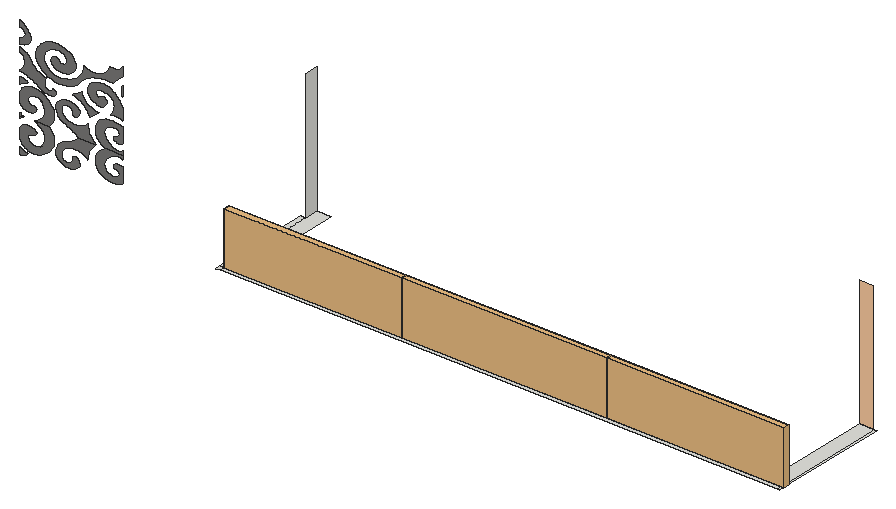
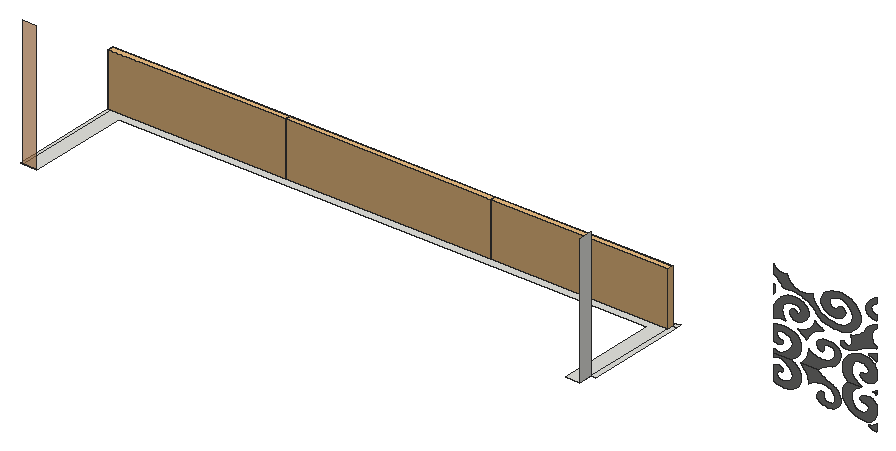
# SketchUp Ruby script. Lengths in inches.
U = 1.inch
M = Sketchup.active_model
def pt(a) = Geom::Point3d.new(a.map { |v| v * U })
def face(e, loops, mat)
  f = e.add_face(loops[0].map { |a| pt(a) })
  loops[1..].each { |l| e.add_face(l.map { |a| pt(a) }).erase! }
  f.material = f.back_material = mat if mat
  f
end
# faces: each face lists its corners as indices into pts; further lists are holes
def faces(e, pts, list, mat = nil) = list.each { |f| face(e, (f[0].is_a?(Array) ? f : [f]).map { |l| l.map { |i| pts[i] } }, mat) }
# xy, xz, yz: faces in a plane at the given z, y or x. An outline is a flat list of corners, or four numbers for a rectangle; further outlines are holes
def ring(l) = l.size == 4 ? [[l[0], l[1]], [l[2], l[1]], [l[2], l[3]], [l[0], l[3]]] : l.each_slice(2).to_a
def flat(e, list, mat, &to3) = list.each { |f| face(e, (f[0].is_a?(Array) ? f : [f]).map { |l| ring(l).map { |u, v| to3.(u, v) } }, mat) }
def xy(e, z, list, mat = nil) = flat(e, list, mat) { |x, y| [x, y, z] }
def xz(e, y, list, mat = nil) = flat(e, list, mat) { |x, z| [x, y, z] }
def yz(e, x, list, mat = nil) = flat(e, list, mat) { |y, z| [x, y, z] }
def lines(e, pts, list) = list.each { |a, b| e.add_line(pt(pts[a]), pt(pts[b])) }
# prism: a flat outline (further loops are holes) pulled along v
def prism(e, loops, v, mat = nil)
  f = face(e, loops, mat); d = Geom::Vector3d.new(v.map { |x| x * U })
  f.pushpull(f.normal.samedirection?(d) ? d.length : -d.length)
end
def box(e, o, s, mat = nil) = prism(e, [[o, [o[0] + s[0], o[1], o[2]], [o[0] + s[0], o[1] + s[1], o[2]], [o[0], o[1] + s[1], o[2]]]], [0, 0, s[2]], mat)
def at(x, y, z, deg = 0) = Geom::Transformation.translation(pt([x, y, z])) * Geom::Transformation.rotation(ORIGIN, Z_AXIS, deg.degrees)
def axes(o, x, y, z) = Geom::Transformation.new([*x, 0, *y, 0, *z, 0, *pt(o).to_a, 1])
def part(name) = M.definitions.add(name)
# library, detail: a bought-in or finely detailed component or shape, given as its bounding box
def library(name, o, s) = part(name).tap { |d| box(d.entities, o, s) }
def detail(e, o, s) = box(e.add_group.entities, o, s)
def put(e, d, t, mat = nil) = e.add_instance(d, t).tap { |i| i.material = mat if mat }
def group(e, t, mat = nil) = e.add_group.tap { |g| g.transformation = t; g.material = mat if mat }.entities
root = M.entities
M.materials.add("[0043_SaddleBrown]4").color = [124, 123, 122]
M.materials.add("[Granite Light Gray]").color = [149, 148, 144]
M.materials.add("[Wood Floor]").color = [224, 152, 88]
M.materials["[Wood Floor]"].alpha = 0.68
c1 = library("Glass Railing",[0,0,0],[139.5,4.76,42])
xy(root,293,[[4300.2,556.4375,4303.63,559.875],[4303.63,556.4375,4742.06,559.875],[4742.06,556.4375,4744,559.875],[4300.2,559.875,4303.63,640.11],[4303.63,559.875,4742.06,559.875,4742.06,651.03,4730.74,651.03,4730.74,571.2,4314.96,571.2,4314.96,651.03,4303.63,651.03],
  [4742.06,559.875,4744,651.03]])
xz(root,589.17,[[4119.85,295.77,4119.85,301,4120.21,300.64,4120.59,300.3,4121.01,299.98,4121.46,299.68,4121.9375,299.4,4122.4375,299.15,4122.96,298.92,4123.51,298.72,4124.07,298.54,4124.64,298.4,4125.23,298.28,4125.83,298.1875,4125.47,297.86,4125.07,297.54,4124.64,297.25,4124.1875,296.98,4123.71,296.74,4123.2,296.52,4122.68,296.32,4122.14,296.15,4121.58,296.02,4121.01,295.91,4120.43,295.82],[4157.82,299.46,4155.83,299.6,4153.91,300.03,4152.16,300.72,4150.64,301.66,4149.42,302.81,4148.55,304.1,4148.05,305.5,4147.91,306.54,4147.89,307.57,4147.99,308.61,4148.22,309.63,4148.57,310.64,4149.05,311.62,4149.64,312.57,4150.34,313.47,4151.15,314.33,4152.06,315.14,4153.06,315.88,4154.16,316.56,4155.31,316.875,4156.43,317.24,4157.53,317.65,4158.59,318.1,4159.62,318.59,4160.6,319.13,4161.55,319.7,4162.44,320.3125,4163.29,320.96,4164.09,321.64,4164.83,322.35,4165.52,323.09,4179.28,323.09,4178.3,322.2,4177.4,321.27,4176.58,320.31,4175.84,319.31,4175.18,318.28,4174.62,317.22,4174.15,316.14,4173.77,315.03,4173.49,313.92,4173.3,312.79,4173.21,311.66,4173.21,310.53,4172.63,311.07,4172,311.58,4171.32,312.0625,4170.59,312.51,4169.83,312.91,4169.02,313.28,4168.18,313.6,4167.3125,313.88,4166.42,314.11,4165.5,314.3,4164.57,314.44,4163.63,314.54,4162,314.5625,4160.39,314.41,4158.83,314.07,4157.37,313.56,4156.03,312.89,4154.86,312.07,4153.88,311.14,4153.12,310.1,4152.59,308.99,4152.31,307.84,4152.28,306.66,4152.52,305.5,4152.77,304.93,4153.16,304.41,4153.68,303.9375,4154.3125,303.54,4155.03,303.24,4155.8125,303.04,4156.63,302.93,4157.46,302.94,4158.28,303.06,4159.05,303.28,4159.76,303.6,4160.37,304,4160.53,304.24,4160.67,304.5,4160.8,304.75,4160.9,305.01,4160.98,305.28,4161.05,305.54,4161.09,305.8125,4161.11,306.08,4161.11,306.36,4161.09,306.625,4161.05,306.9,4160.99,307.16,4160.96,307.41,4160.98,307.66,4161.07,307.9,4161.21,308.13,4161.4,308.34,4161.64,308.52,4161.92,308.67,4162.23,308.78,4162.56,308.85,4162.9,308.875,4163.25,308.86,4163.58,308.8,4164.19,308.46,4164.74,308.07,4165.23,307.64,4165.65,307.17,4166,306.68,4166.27,306.15,4166.46,305.61,4166.57,305.0625,4166.59,304.51,4166.53,303.95,4166.39,303.41,4166.16,302.875,4164.96,301.72,4163.45,300.77,4161.71,300.06,4159.81,299.61],[4130.68,299.94,4129.11,299.97,4127.57,300.16,4126.08,300.52,4124.68,301.04,4123.41,301.7,4122.3,302.5,4121.37,303.41,4120.64,304.41,4120.13,305.48,4119.85,306.59,4119.85,314.54,4120.3125,315.41,4120.99,316.19,4121.86,316.875,4122.9,317.42,4124.06,317.82,4125.3,318.05,4126.58,318.11,4127.86,318,4129.08,317.71,4130.21,317.27,4131.19,316.67,4132.01,315.96,4132.25,315.64,4132.41,315.29,4132.48,314.93,4132.46,314.57,4132.34,314.22,4132.14,313.88,4131.86,313.58,4131.51,313.32,4131.1,313.11,4130.64,312.96,4130.16,312.86,4129.65,312.84,4128.99,312.8,4128.34,312.6875,4127.73,312.49,4127.18,312.23,4126.69,311.89,4126.3,311.51,4126,311.08,4125.81,310.62,4125.73,310.14,4125.77,309.66,4125.92,309.1875,4126.19,308.75,4126.57,307.98,4127.14,307.28,4127.89,306.67,4128.78,306.17,4129.78,305.8,4130.87,305.58,4131.99,305.5,4133.11,305.58,4134.2,305.81,4135.2,306.18,4136.62,307.48,4137.75,308.92,4138.56,310.46,4139.04,312.08,4139.16,313.73,4138.9375,315.38,4138.36,316.98,4137.46,318.5,4136.24,319.9,4134.74,321.15,4132.99,322.22,4131.04,323.09,4141.98,323.09,4143.81,321.23,4145.2,319.18,4146.14,317,4146.58,314.75,4146.52,312.47,4145.96,310.22,4144.92,308.07,4143.42,306.0625,4141.5,304.25,4139.21,302.68,4136.6,301.39,4133.74,300.42,4132.24,300.1],[4192.52,301.35,4189.81,301.57,4187.22,302.17,4184.85,303.12,4182.78,304.39,4181.09,305.93,4179.86,307.67,4179.13,309.5625,4178.93,311.52,4179.27,313.46,4179.35,314.46,4179.56,315.44,4179.88,316.41,4180.33,317.35,4180.9,318.26,4181.58,319.125,4182.37,319.94,4183.26,320.71,4184.24,321.41,4185.3,322.04,4186.44,322.6,4187.65,323.09,4200.24,323.09,4200.24,320.125,4199.94,320.4,4199.6,320.65,4199.21,320.87,4198.8,321.05,4198.36,321.2,4197.89,321.3,4197.42,321.37,4196.93,321.4,4196.44,321.38,4195.96,321.32,4195.5,321.23,4195.05,321.09,4193.97,320.67,4192.93,320.19,4191.95,319.66,4191.02,319.08,4190.15,318.45,4189.35,317.78,4188.62,317.07,4187.95,316.33,4187.37,315.55,4186.87,314.74,4186.44,313.91,4186.1,313.06,4185.91,312.23,4185.875,311.39,4186.02,310.55,4186.32,309.74,4186.79,308.97,4187.4,308.25,4188.15,307.61,4189.03,307.05,4190.01,306.59,4191.0625,306.24,4192.18,306,4193.34,305.875,4194.4,305.92,4195.42,306.14,4196.33,306.54,4197.08,307.09,4197.62,307.75,4197.92,308.49,4197.96,309.26,4197.74,310.01,4197.27,310.7,4196.58,311.28,4195.71,311.73,4194.72,312.01,4194.48,312,4194.23,312.01,4193.99,312.06,4193.77,312.13,4193.5625,312.23,4193.39,312.36,4193.24,312.5,4193.14,312.66,4193.07,312.83,4193.04,313.01,4193.06,313.18,4193.12,313.36,4193.4,313.84,4193.79,314.28,4194.28,314.67,4194.84,315,4195.47,315.25,4196.16,315.43,4196.87,315.53,4197.6,315.54,4198.3125,315.47,4199.01,315.3125,4199.65,315.08,4200.24,314.77,4200.24,302.99,4197.83,302.08,4195.23,301.53],[4119.85,321.36,4119.85,323.09,4122.25,323.09,4121.93,323.07,4121.63,323.03,4121.33,322.96,4121.05,322.86,4120.79,322.73,4120.55,322.58,4120.35,322.41,4120.17,322.22,4120.03,322.02,4119.93,321.81,4119.87,321.59],
  [4119.85,323.09,4122.25,323.09,4121.93,323.1,4121.63,323.15,4121.33,323.22,4121.05,323.32,4120.79,323.45,4120.55,323.59,4120.35,323.76,4120.17,323.95,4120.03,324.16,4119.93,324.37,4119.87,324.59,4119.85,324.82],[4131.04,323.09,4141.98,323.09,4143.81,324.95,4145.2,326.99,4146.14,329.17,4146.58,331.43,4146.52,333.71,4145.96,335.95,4144.92,338.11,4143.42,340.11,4141.5,341.93,4139.21,343.5,4136.6,344.78,4133.74,345.76,4132.24,346.08,4130.68,346.23,4129.11,346.21,4127.57,346.02,4126.08,345.66,4124.68,345.14,4123.41,344.47,4122.3,343.68,4121.37,342.77,4120.64,341.77,4120.13,340.7,4119.85,339.58,4119.85,331.63,4120.3125,330.77,4120.99,329.98,4121.86,329.3,4122.9,328.75,4124.06,328.36,4125.3,328.12,4126.58,328.0625,4127.86,328.18,4129.08,328.46,4130.21,328.91,4131.19,329.5,4132.01,330.22,4132.25,330.54,4132.41,330.88,4132.48,331.24,4132.46,331.61,4132.34,331.96,4132.14,332.29,4131.86,332.6,4131.51,332.86,4131.1,333.07,4130.64,333.22,4130.16,333.3125,4129.65,333.34,4128.99,333.375,4128.34,333.49,4127.73,333.68,4127.18,333.95,4126.69,334.28,4126.3,334.67,4126,335.1,4125.81,335.5625,4125.73,336.04,4125.77,336.52,4125.92,336.99,4126.19,337.43,4126.57,338.2,4127.14,338.9,4127.89,339.51,4128.78,340,4129.78,340.375,4130.87,340.6,4131.99,340.68,4133.11,340.6,4134.2,340.37,4135.2,340,4136.62,338.7,4137.75,337.26,4138.56,335.71,4139.04,334.1,4139.16,332.44,4138.9375,330.8,4138.36,329.2,4137.46,327.68,4136.24,326.28,4134.74,325.02,4132.99,323.95],[4165.52,323.09,4179.28,323.09,4178.3,323.97,4177.4,324.9,4176.58,325.87,4175.84,326.87,4175.18,327.9,4174.62,328.96,4174.15,330.04,4173.77,331.14,4173.49,332.26,4173.3,333.38,4173.21,334.51,4173.21,335.65,4172.63,335.11,4172,334.59,4171.32,334.11,4170.59,333.67,4169.83,333.27,4169.02,332.9,4168.18,332.58,4167.3125,332.3,4166.42,332.0625,4165.5,331.875,4164.57,331.73,4163.63,331.64,4162,331.61,4160.39,331.77,4158.83,332.11,4157.37,332.62,4156.03,333.29,4154.86,334.1,4153.88,335.04,4153.12,336.08,4152.59,337.18,4152.31,338.34,4152.28,339.51,4152.52,340.67,4152.77,341.24,4153.16,341.77,4153.68,342.24,4154.3125,342.63,4155.03,342.9375,4155.8125,343.14,4156.63,343.24,4157.46,343.23,4158.28,343.12,4159.05,342.9,4159.76,342.58,4160.37,342.18,4160.53,341.93,4160.67,341.68,4160.8,341.42,4160.9,341.16,4160.98,340.9,4161.05,340.63,4161.09,340.36,4161.11,340.09,4161.11,339.82,4161.09,339.55,4161.05,339.28,4160.99,339.01,4160.96,338.76,4160.98,338.52,4161.07,338.27,4161.21,338.05,4161.4,337.84,4161.64,337.66,4161.92,337.51,4162.23,337.4,4162.56,337.33,4162.9,337.3,4163.25,337.32,4163.58,337.37,4164.19,337.72,4164.74,338.11,4165.23,338.54,4165.65,339,4166,339.5,4166.27,340.02,4166.46,340.5625,4166.57,341.11,4166.59,341.67,4166.53,342.22,4166.39,342.77,4166.16,343.3,4164.96,344.45,4163.45,345.41,4161.71,346.12,4159.81,346.5625,4157.82,346.72,4155.83,346.58,4153.91,346.15,4152.16,345.45,4150.64,344.51,4149.42,343.37,4148.55,342.07,4148.05,340.67,4147.91,339.64,4147.89,338.6,4147.99,337.57,4148.22,336.54,4148.57,335.54,4149.05,334.56,4149.64,333.61,4150.34,332.7,4151.15,331.84,4152.06,331.04,4153.06,330.3,4154.16,329.62,4155.31,329.3,4156.43,328.9375,4157.53,328.53,4158.59,328.08,4159.62,327.58,4160.6,327.05,4161.55,326.47,4162.44,325.86,4163.29,325.22,4164.09,324.54,4164.83,323.83],[4187.65,323.09,4200.24,323.09,4200.24,326.05,4199.94,325.77,4199.6,325.53,4199.21,325.31,4198.8,325.125,4198.36,324.98,4197.89,324.87,4197.42,324.8,4196.93,324.78,4196.44,324.79,4195.96,324.85,4195.5,324.95,4195.05,325.09,4193.97,325.51,4192.93,325.99,4191.95,326.52,4191.02,327.1,4190.15,327.72,4189.35,328.39,4188.62,329.1,4187.95,329.85,4187.37,330.625,4186.87,331.43,4186.44,332.27,4186.1,333.12,4185.91,333.95,4185.875,334.79,4186.02,335.62,4186.32,336.44,4186.79,337.21,4187.4,337.92,4188.15,338.57,4189.03,339.125,4190.01,339.58,4191.0625,339.9375,4192.18,340.18,4193.34,340.3,4194.4,340.26,4195.42,340.03,4196.33,339.64,4197.08,339.09,4197.62,338.43,4197.92,337.6875,4197.96,336.92,4197.74,336.17,4197.27,335.48,4196.58,334.89,4195.71,334.45,4194.72,334.17,4194.48,334.18,4194.23,334.17,4193.99,334.12,4193.77,334.05,4193.5625,333.95,4193.39,333.82,4193.24,333.68,4193.14,333.52,4193.07,333.35,4193.04,333.17,4193.06,332.99,4193.12,332.82,4193.4,332.34,4193.79,331.9,4194.28,331.51,4194.84,331.18,4195.47,330.92,4196.16,330.74,4196.87,330.65,4197.6,330.64,4198.3125,330.71,4199.01,330.86,4199.65,331.1,4200.24,331.41,4200.24,343.1875,4197.83,344.1,4195.23,344.65,4192.52,344.82,4189.81,344.61,4187.22,344.01,4184.85,343.06,4182.78,341.79,4181.09,340.25,4179.86,338.5,4179.13,336.61,4178.93,334.66,4179.27,332.71,4179.35,331.72,4179.56,330.74,4179.88,329.77,4180.33,328.83,4180.9,327.92,4181.58,327.05,4182.37,326.23,4183.26,325.47,4184.24,324.77,4185.3,324.13,4186.44,323.57],[4174.41,341.21,4174.94,341.68,4175.48,342.15,4176.03,342.61,4176.59,343.0625,4177.16,343.51,4177.75,343.95,4178.34,344.38,4178.9375,344.81,4179.55,345.23,4180.17,345.64,4180.8,346.04,4181.4375,346.4375,4179.77,346.72,4178.15,347.12,4176.61,347.65,4175.15,348.29,4173.8,349.05,4172.5625,349.9,4171.46,350.85,4170.51,351.87,4169.72,352.97,4169.09,354.11,4168.64,355.3,4168.37,356.52,4167.82,356.14,4167.26,355.77,4166.69,355.4,4166.12,355.04,4165.53,354.69,4164.9375,354.35,4164.34,354.02,4163.72,353.6875,4163.11,353.37,4161.85,352.75,4161.2,352.46,4162.81,351.92,4164.35,351.3,4165.8125,350.58,4167.2,349.79,4168.49,348.92,4169.6875,347.98,4170.77,346.98,4171.75,345.91,4172.61,344.8,4173.34,343.64,4173.94,342.4375],
  [4119.85,345.18,4120.21,345.53,4120.59,345.875,4121.01,346.2,4121.46,346.5,4121.9375,346.77,4122.4375,347.03,4122.96,347.26,4123.51,347.46,4124.07,347.63,4124.64,347.78,4125.23,347.9,4125.83,347.99,4125.47,348.32,4125.07,348.63,4124.64,348.93,4124.1875,349.19,4123.71,349.44,4123.2,349.66,4122.68,349.85,4122.14,350.02,4121.58,350.16,4121.01,350.27,4120.43,350.35,4119.85,350.4],[4143.5,345.8,4144.51,345.82,4145.33,345.91,4146.09,346.14,4146.77,346.49,4147.3125,346.93,4147.71,347.45,4147.93,348.03,4147.97,348.625,4147.82,349.21,4147.49,349.76,4147,350.24,4146.375,350.625,4145.64,350.9,4145.53,350.3,4145.21,349.75,4144.71,349.27,4144.04,348.9,4143.27,348.67,4142.44,348.59,4141.61,348.67,4140.84,348.9,4140.18,349.27,4139.67,349.75,4139.35,350.3,4139.24,350.9,4139.2,351.375,4139.17,351.85,4139.16,352.33,4139.17,352.8,4139.2,353.28,4139.24,353.75,4139.3,354.22,4139.38,354.7,4139.48,355.17,4139.6,355.63,4139.73,356.1,4139.88,356.5625,4138.42,356.99,4137,357.49,4135.65,358.08,4134.37,358.74,4133.16,359.47,4132.04,360.27,4131.01,361.14,4130.08,362.05,4129.25,363.02,4128.53,364.03,4127.93,365.09,4127.44,366.17,4126.92,366.67,4126.37,367.16,4125.8,367.64,4125.22,368.1,4124.61,368.55,4123.98,368.99,4123.34,369.41,4122.67,369.82,4121.99,370.21,4121.29,370.59,4120.58,370.95,4119.85,371.29,4119.85,368.08,4120.87,367.17,4121.73,366.18,4122.41,365.12,4122.9,364.01,4123.2,362.86,4123.3,361.69,4123.2,360.52,4122.9,359.375,4122.41,358.26,4121.73,357.2,4120.87,356.21,4119.85,355.3,4119.85,354.25,4121.14,354.05,4122.41,353.81,4123.66,353.53,4124.89,353.19,4126.1,352.8125,4127.27,352.39,4128.41,351.92,4129.52,351.4,4130.58,350.85,4131.61,350.26,4132.59,349.63,4133.53,348.96,4134.25,348.45,4135.03,347.98,4135.85,347.55,4136.72,347.16,4137.61,346.82,4138.54,346.53,4139.5,346.28,4140.48,346.08,4141.48,345.9375,4142.48,345.85],[4200.24,347.78,4200.24,356.71,4199.875,357.36,4199.5,358,4199.1,358.64,4198.6875,359.27,4198.26,359.9,4197.82,360.52,4197.36,361.13,4196.89,361.74,4196.41,362.35,4195.9,362.95,4195.39,363.54,4194.86,364.12,4194,364.94,4193.02,365.6875,4191.92,366.34,4190.73,366.9,4189.45,367.36,4188.11,367.71,4186.73,367.94,4185.3125,368.0625,4183.89,368.0625,4182.47,367.94,4181.09,367.71,4179.75,367.36,4177.8125,366.59,4176.12,365.57,4174.73,364.33,4173.7,362.92,4173.07,361.39,4172.85,359.81,4173.07,358.23,4173.7,356.7,4174.73,355.29,4176.12,354.05,4177.8125,353.03,4179.75,352.26,4180.39,351.99,4181.08,351.8,4181.81,351.6875,4182.55,351.66,4183.29,351.71,4184.01,351.86,4184.68,352.08,4185.3,352.37,4185.85,352.73,4186.3125,353.15,4186.68,353.62,4186.93,354.12,4187.3,354.57,4187.57,355.05,4187.75,355.55,4187.83,356.0625,4187.8,356.58,4187.68,357.09,4187.45,357.59,4187.13,358.05,4186.73,358.48,4186.24,358.86,4185.6875,359.19,4185.07,359.46,4184.72,359.32,4184.38,359.17,4184.05,359,4183.74,358.82,4183.45,358.62,4183.18,358.41,4182.93,358.18,4182.7,357.94,4182.5,357.69,4182.32,357.43,4182.16,357.17,4182.04,356.89,4181.27,357.23,4180.6,357.65,4180.06,358.17,4179.66,358.74,4179.41,359.36,4179.33,360,4179.41,360.64,4179.66,361.26,4180.06,361.84,4180.6,362.35,4181.27,362.78,4182.04,363.11,4182.97,363.13,4183.9,363.11,4184.83,363.03,4185.75,362.91,4186.65,362.73,4187.53,362.51,4188.39,362.24,4189.21,361.93,4190,361.57,4190.76,361.17,4191.47,360.73,4192.13,360.26,4192.71,359.34,4193.18,358.39,4193.53,357.41,4193.75,356.41,4193.85,355.41,4193.82,354.4,4193.67,353.39,4193.39,352.4,4192.99,351.4375,4192.47,350.5,4191.83,349.6,4191.09,348.74,4191.85,348.93,4192.63,349.07,4193.43,349.17,4194.23,349.21,4195.04,349.2,4195.84,349.14,4196.63,349.03,4197.41,348.875,4198.16,348.67,4198.89,348.42,4199.59,348.12],[4150.52,356.35,4153.68,356.47,4156.77,356.98,4159.6875,357.86,4162.36,359.07,4164.71,360.6,4166.67,362.39,4167.21,363.14,4167.8,363.86,4168.43,364.5625,4169.12,365.25,4169.84,365.9,4170.61,366.53,4171.42,367.14,4172.26,367.72,4173.15,368.26,4174.07,368.78,4175.02,369.26,4176,369.72,4177.3,370.16,4178.64,370.56,4180,370.9,4181.39,371.18,4182.79,371.41,4184.21,371.59,4185.65,371.7,4187.09,371.76,4188.53,371.77,4189.97,371.71,4191.4,371.6,4192.83,371.43,4193.38,372.07,4193.95,372.71,4194.53,373.34,4195.12,373.96,4195.72,374.58,4196.33,375.19,4196.96,375.8,4197.59,376.4,4198.24,376.99,4198.9,377.58,4199.5625,378.16,4200.24,378.74,4200.24,385.48,4199.875,384.78,4199.375,384.13,4198.76,383.54,4198.03,383.01,4197.2,382.5625,4196.3,382.2,4195.34,381.9375,4194.33,381.77,4193.3,381.71,4192.27,381.75,4191.26,381.9,4190.28,382.14,4189.84,380.54,4189.03,379.02,4187.86,377.62,4186.38,376.38,4184.63,375.35,4182.66,374.54,4180.53,373.99,4178.3,373.7,4176.04,373.7,4173.8,373.98,4171.67,374.52,4169.7,375.32,4169.63,373.3,4169.17,371.31,4168.3,369.39,4167.0625,367.57,4165.47,365.91,4163.56,364.43,4161.37,363.17,4158.95,362.14,4156.35,361.39,4153.63,360.91,4150.84,360.72,4148.04,360.82,4145.59,361.55,4143.37,362.6,4141.48,363.94,4139.99,365.52,4138.94,367.27,4138.39,369.14,4138.34,371.05,4138.8125,372.94,4139.78,374.72,4141.2,376.33,4143.02,377.71,4145.1875,378.82,4146.58,379.26,4148.07,379.49,4149.6,379.5,4151.09,379.28,4152.49,378.85,4153.75,378.22,4154.79,377.42,4155.59,376.48,4156.11,375.45,4156.32,374.36,4156.22,373.26,4155.81,372.2,4155.54,371.81,4155.16,371.47,4154.7,371.19,4154.16,370.98,4153.59,370.85,4152.98,370.81,4152.38,370.85,4151.8,370.98,4151.27,371.19,4150.8,371.47,4150.43,371.81,4150.15,372.2,4150.01,372.43,4149.85,372.65,4149.66,372.85,4149.45,373.05,4149.22,373.23,4148.97,373.4,4148.71,373.55,4148.42,373.6875,4148.12,373.81,4147.81,373.91,4147.49,373.99,4147.16,374.05,4146.58,373.81,4146.04,373.51,4145.56,373.17,4145.14,372.79,4144.79,372.37,4144.51,371.93,4144.31,371.47,4144.1875,370.99,4144.15,370.5,4144.19,370.02,4144.32,369.54,4144.52,369.08,4144.91,368.45,4145.39,367.87,4145.96,367.32,4146.6,366.82,4147.32,366.37,4148.09,365.98,4148.92,365.65,4149.8,365.39,4150.7,365.2,4151.63,365.08,4152.58,365.03,4153.52,365.05,4155.02,365.22,4156.46,365.53,4157.84,365.98,4159.12,366.56,4160.29,367.25,4161.31,368.05,4162.18,368.95,4162.87,369.91,4163.38,370.9375,4163.7,372,4163.8125,373.09,4163.73,374.18,4163.12,375.81,4162.2,377.37,4160.98,378.8125,4159.49,380.12,4157.75,381.26,4155.8125,382.21,4153.7,382.95,4151.47,383.47,4149.16,383.76,4146.8125,383.8,4144.48,383.61,4142.21,383.18,4140.02,382.09,4138.03,380.8125,4136.3,379.36,4134.84,377.75,4133.68,376.03,4132.84,374.21,4132.34,372.32,4132.17,370.41,4132.35,368.5,4132.88,366.62,4133.74,364.8,4134.91,363.08,4136.72,361.21,4138.94,359.58,4141.5,358.25,4144.35,357.25,4147.38,356.61],[4200.24,364.66,4200.24,371.94,4200.02,371.35,4199.83,370.75,4199.6875,370.14,4199.58,369.53,4199.52,368.92,4199.5,368.3,4199.52,367.69,4199.58,367.07,4199.6875,366.46,4199.83,365.85,4200.02,365.25],
  [4119.85,373.83,4121.1,373.9,4122.32,374.11,4123.48,374.45,4124.56,374.91,4125.52,375.49,4126.36,376.16,4127.04,376.92,4127.5625,377.74,4127.9,378.61,4128.05,379.51,4128.01,380.41,4127.79,381.3,4127.4375,382.16,4127.03,383.01,4126.55,383.84,4126.02,384.65,4125.43,385.45,4124.79,386.22,4124.09,386.96,4123.34,387.68,4122.54,388.36,4121.6875,389.02,4120.79,389.64,4119.85,390.23,4119.85,385.49,4120.93,385.16,4121.9,384.67,4122.7,384.05,4123.3,383.32,4123.67,382.52,4123.79,381.67,4123.67,380.83,4123.3,380.02,4122.7,379.29,4121.9,378.67,4120.93,378.18,4119.85,377.85]],"[0043_SaddleBrown]4")
xz(root,651.03,[[4730.74,293,4742.06,394.4375]],"[Wood Floor]")
yz(root,4303.63,[[640.11,293,651.03,394.4375]])
p = [[4135.2,589.17,306.18],[4136.09,589.17,306.68],[4136.83,589.17,307.29],[4135.2,589.17,340],[4136.09,589.17,339.5],[4136.83,589.17,338.89]]
lines(root,p,[[0,1],[1,2],[3,4],[4,5]])
put(root,c1,at(4303.63,559.875,293))
put(root,c1,axes([4443.13,559.875,293],[1.15726,0,0],[0,1,0],[0,0,1]),"[Granite Light Gray]")
put(root,c1,at(4604.57,559.875,293))
